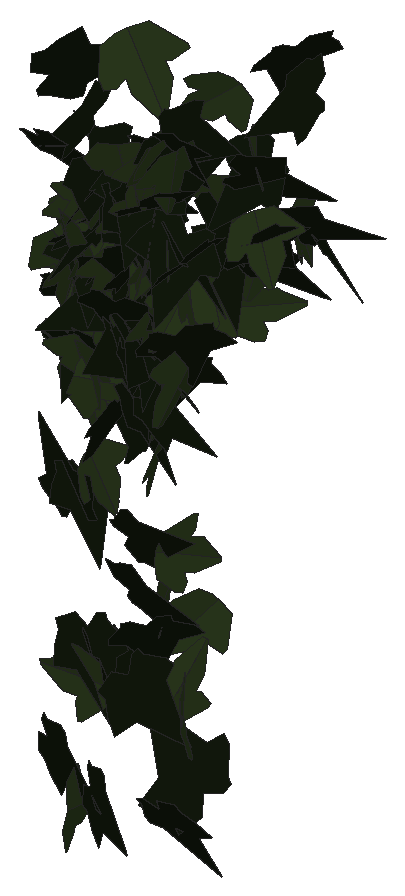
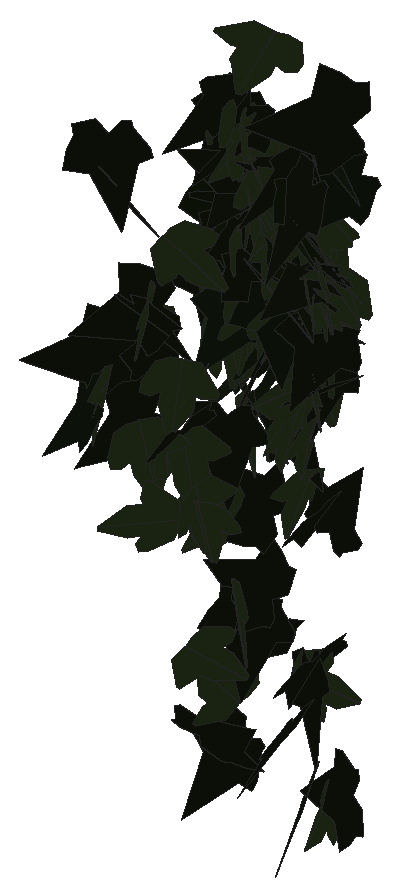
# SketchUp Ruby script. Lengths in inches.
U = 1.inch
M = Sketchup.active_model
def pt(a) = Geom::Point3d.new(a.map { |v| v * U })
def face(e, loops, mat)
  f = e.add_face(loops[0].map { |a| pt(a) })
  loops[1..].each { |l| e.add_face(l.map { |a| pt(a) }).erase! }
  f.material = f.back_material = mat if mat
  f
end
# faces: each face lists its corners as indices into pts; further lists are holes
def faces(e, pts, list, mat = nil) = list.each { |f| face(e, (f[0].is_a?(Array) ? f : [f]).map { |l| l.map { |i| pts[i] } }, mat) }
# xy, xz, yz: faces in a plane at the given z, y or x. An outline is a flat list of corners, or four numbers for a rectangle; further outlines are holes
def ring(l) = l.size == 4 ? [[l[0], l[1]], [l[2], l[1]], [l[2], l[3]], [l[0], l[3]]] : l.each_slice(2).to_a
def flat(e, list, mat, &to3) = list.each { |f| face(e, (f[0].is_a?(Array) ? f : [f]).map { |l| ring(l).map { |u, v| to3.(u, v) } }, mat) }
def xy(e, z, list, mat = nil) = flat(e, list, mat) { |x, y| [x, y, z] }
def xz(e, y, list, mat = nil) = flat(e, list, mat) { |x, z| [x, y, z] }
def yz(e, x, list, mat = nil) = flat(e, list, mat) { |y, z| [x, y, z] }
def lines(e, pts, list) = list.each { |a, b| e.add_line(pt(pts[a]), pt(pts[b])) }
# prism: a flat outline (further loops are holes) pulled along v
def prism(e, loops, v, mat = nil)
  f = face(e, loops, mat); d = Geom::Vector3d.new(v.map { |x| x * U })
  f.pushpull(f.normal.samedirection?(d) ? d.length : -d.length)
end
def box(e, o, s, mat = nil) = prism(e, [[o, [o[0] + s[0], o[1], o[2]], [o[0] + s[0], o[1] + s[1], o[2]], [o[0], o[1] + s[1], o[2]]]], [0, 0, s[2]], mat)
def at(x, y, z, deg = 0) = Geom::Transformation.translation(pt([x, y, z])) * Geom::Transformation.rotation(ORIGIN, Z_AXIS, deg.degrees)
def axes(o, x, y, z) = Geom::Transformation.new([*x, 0, *y, 0, *z, 0, *pt(o).to_a, 1])
def part(name) = M.definitions.add(name)
# library, detail: a bought-in or finely detailed component or shape, given as its bounding box
def library(name, o, s) = part(name).tap { |d| box(d.entities, o, s) }
def detail(e, o, s) = box(e.add_group.entities, o, s)
def put(e, d, t, mat = nil) = e.add_instance(d, t).tap { |i| i.material = mat if mat }
def group(e, t, mat = nil) = e.add_group.tap { |g| g.transformation = t; g.material = mat if mat }.entities
root = M.entities
M.materials.add("efeu1").color = [18, 25, 13]
M.materials.add("efeu2").color = [43, 57, 29]
c1 = part("ivyleaf_9")
p = [[1.54,2.16,1.25],[1.36,2.04,1.19],[-0.21,0.99,0.68],[-0.71,1.11,0.82],[-0.85,0.86,0.67],[-0.8,0.17,0.21],
  [-0.9,-0.01,0.1],[-0.67,-0.16,-0.02],[-0.08,-0.08,-0.05],[-0.03,-0.6,-0.4],[0.65,-0.88,-0.66],[0.83,-0.6,-0.49],
  [1.29,-0.42,-0.43],[1.8125,-0.07,-0.26],[1.21,0.44,0.15]]
faces(c1.entities,p,[[0,1,2,3,4,5,6,7,8,9,10,11,12,13,14]],"efeu1")
c2 = part("ivyleaf_10")
p = [[0,0.5,-0.03],[-0.0625,2.02,-0.43],[-0.19,2.01,-0.46],[-0.54,1.05,-0.29],[-0.52,0.625,-0.18],[-0.83,0.76,-0.28],
  [-1.16,0.64,-0.33],[-1.15,0.33,-0.24],[-0.77,-0.39,0.02],[-0.3,-0.51,0.16],[0.04,-0.48,0.23],[-0.02,2.01,-0.4375],
  [-0.06,2.01,-0.43],[0.04,-0.49,0.23],[0.67,-0.49,0.14],[1.38,0.36,-0.2],[1.375,0.51,-0.24],[0.81,0.65,-0.19],
  [0.62,0.59,-0.15],[0.6,1.09,-0.28],[0.5,1.23,-0.31]]
faces(c2.entities,p,[[0,1,2,3,4,5,6,7,8,9,10],[11,12,0,13,14,15,16,17,18,19,20]],"efeu2")
put(root,c1,axes([544.76,134.72,188.62],[0.26461,-0.49015,-0.62261],[-0.11295,0.62638,-0.54111],[0.7843,0.25557,0.13213]))
put(root,c1,axes([544.53,135.6,197.67],[-0.09645,-0.52638,0.59874],[0.11267,-0.60605,-0.51465],[0.78922,0.02219,0.14664]))
put(root,c1,axes([545.9,135.43,201.21],[-0.46865,-0.66084,-0.06581],[0.07755,0.02553,-0.80871],[0.65957,-0.47256,0.04833]))
put(root,c2,axes([543.35,135.14,201.56],[-0.61815,-0.37302,0.40934],[-0.34419,-0.22182,-0.7219],[0.43386,-0.70743,0.01051]))
put(root,c2,axes([543.34,134.95,187.91],[0.05962,-0.02944,-0.83382],[-0.8038,0.22209,-0.06531],[0.22369,0.80591,-0.01246]))
put(root,c1,axes([544.24,134.74,199.09],[0.5135,0.45053,-0.41731],[-0.39056,-0.1802,-0.67513],[-0.47391,0.63668,0.10421]))
put(root,c1,axes([545.73,134.73,185.15],[0.85129,0.12056,-0.12346],[-0.12249,-0.01554,-0.85979],[-0.12154,0.86006,0.00177]))
put(root,c2,axes([545.02,135.13,200.87],[0.77564,-0.25844,-0.09532],[-0.09055,0.02979,-0.81756],[0.26015,0.78091,-0.00036]))
put(root,c2,axes([543.06,135.12,197.1],[-0.62944,-0.37013,0.31975],[-0.27822,-0.15765,-0.73019],[0.40228,-0.68817,-0.0047]))
put(root,c1,axes([543.95,135.68,197.38],[0.32213,-0.46197,-0.56698],[0.30459,-0.47851,0.56294],[-0.66491,-0.44302,-0.01681]))
put(root,c2,axes([545.8,135.56,197.49],[0.11949,-0.7861,0.55869],[0.12562,-0.54548,-0.79438],[0.95619,0.1699,0.03454]))
put(root,c2,axes([545.8,135.11,203.51],[-0.11866,-0.8194,-0.02635],[0.01545,0.02439,-0.82787],[0.81968,-0.11908,0.01179]))
put(root,c2,axes([544.25,134.98,203.22],[-0.69949,-0.4216,-0.0796],[0.0593,0.05578,-0.81655],[0.42494,-0.7018,-0.01708]))
put(root,c2,axes([543,134.97,197.16],[-0.72287,0.30848,-0.06623],[0.05691,-0.03537,-0.78587],[-0.31034,-0.72504,0.01016]))
put(root,c2,axes([542.57,134.92,200.67],[-0.74013,0.35899,0.06304],[-0.05424,0.03261,-0.82258],[-0.36042,-0.74209,-0.00565]))
put(root,c2,axes([544.97,135.35,203.03],[-0.15827,-0.75081,0.27557],[-0.01987,-0.27714,-0.76649],[0.79954,-0.15551,0.0355]))
put(root,c1,axes([543.5,135.375,201.18],[-0.68086,0.24372,-0.34248],[0.24183,-0.30612,-0.69862],[-0.34382,-0.69796,0.18682]))
put(root,c1,axes([544.46,135.12,192.33],[0.6246,0.15303,-0.47673],[0.43965,0.19707,0.63928],[0.23958,-0.76063,0.06972]))
put(root,c1,axes([546.18,134.77,198.79],[0.42333,0.69725,-0.21629],[-0.10931,-0.18667,-0.81569],[-0.72179,0.4372,-0.00333]))
put(root,c2,axes([544.79,135.5625,201.25],[-0.20567,0.32932,-0.7003],[0.18555,-0.68249,-0.37544],[-0.75129,-0.25871,0.09899]))
put(root,c2,axes([545,135.23,203.39],[0.21388,-0.79503,0.01086],[0.01094,-0.0083,-0.82325],[0.79503,0.21399,0.00841]))
put(root,c2,axes([542.95,134.57,184.39],[0.09931,-0.29894,-0.80701],[-0.04553,0.8094,-0.30543],[0.8594,0.07743,0.07707]))
put(root,c1,axes([543.23,135.03,203.92],[-0.55428,0.61063,0.06662],[-0.09364,0.00469,-0.82204],[-0.60708,-0.55825,0.06596]))
put(root,c1,axes([544.67,135.52,202.45],[-0.48451,-0.62371,-0.1688],[0.13918,0.10529,-0.78854],[0.63098,-0.50215,0.04433]))
put(root,c1,axes([541.84,134.87,202.86],[0.8272,0.06653,-0.0089],[-0.01473,0.07252,-0.82661],[-0.06549,0.82406,0.07346]))
put(root,c2,axes([544.58,135.11,201.8],[-0.3463,-0.70029,-0.17635],[0.10079,0.1468,-0.78085],[0.71509,-0.35982,0.02465]))
put(root,c1,axes([544.1875,135.39,201.78],[0.26114,-0.7518,-0.13057],[-0.05401,0.11945,-0.79578],[0.76114,0.26641,-0.01167]))
put(root,c2,axes([543.8,135.39,199.96],[-0.18823,-0.77605,0.16166],[-0.03684,-0.15741,-0.79855],[0.79185,-0.1918,0.00128]))
put(root,c2,axes([544.62,135.24,200.5],[0.55391,-0.56546,-0.20766],[-0.1416,0.15197,-0.79154],[0.5855,0.5717,0.00502]))
put(root,c1,axes([542.5625,134.99,197.46],[0.66487,0.22568,-0.35782],[-0.33337,-0.13085,-0.70197],[-0.26044,0.74361,-0.01492]))
put(root,c2,axes([545.88,135.46,199.6],[0.46267,0.52111,-0.41546],[-0.28247,-0.30476,-0.69682],[-0.60363,0.54203,0.00764]))
put(root,c1,axes([542.46,135.18,192.63],[0.39249,-0.24506,0.67965],[-0.43984,0.53257,0.44603],[-0.57317,-0.5765,0.12313]))
put(root,c1,axes([543.84,134.82,200.17],[0.61538,0.5123,0.01662],[0.0124,0.01108,-0.80071],[-0.51242,0.6155,0.00058]))
put(root,c1,axes([544.33,135.39,196.07],[0.5133,-0.61052,0.01301],[0.00313,-0.01437,-0.7976],[0.61065,0.51326,-0.00685]))
put(root,c1,axes([543.28,135.01,184.8],[0.50992,-0.33187,-0.57273],[-0.48933,0.29789,-0.60828],[0.44578,0.70662,-0.01256]))
put(root,c1,axes([544.98,135.55,198.59],[-0.59767,-0.19423,-0.50469],[0.50881,0.0528,-0.62288],[0.18316,-0.78047,0.08346]))
put(root,c1,axes([542.59,135.55,193.17],[0.14743,-0.7677,-0.05262],[0.00797,0.0551,-0.78152],[0.76946,0.14653,0.01818]))
put(root,c2,axes([543.52,135.33,201.78],[-0.06262,-0.81239,-0.06941],[-0.0248,0.07148,-0.81424],[0.81497,-0.06024,-0.03012]))
put(root,c1,axes([543.46,135.09,201.9375],[-0.26081,0.76593,-0.10414],[0.04542,-0.09454,-0.80902],[-0.77164,-0.26444,-0.01242]))
put(root,c1,axes([545.07,135,196.48],[0.68894,-0.28627,-0.37646],[-0.20713,0.41535,-0.69491],[0.42517,0.66622,0.27147]))
put(root,c1,axes([541.54,135.51,185.375],[0.15811,0.00107,-0.85529],[0.84517,0.13322,0.15641],[0.1312,-0.85952,0.02318]))
put(root,c1,axes([544.27,135.34,199.3],[-0.15862,-0.08005,-0.94213],[-0.87716,-0.3442,0.17693],[-0.35301,0.89123,-0.01629]))
put(root,c2,axes([542.81,135.45,201.24],[-0.45591,-0.66819,0.06412],[0.04088,-0.105,-0.80359],[0.67002,-0.44826,0.09265]))
put(root,c2,axes([545.1,135.41,195.11],[0.36867,-0.7287,-0.08806],[-0.03604,0.08045,-0.81664],[0.73311,0.3704,0.00414]))
put(root,c2,axes([545.31,135.34,203.62],[-0.02715,-0.80702,-0.12925],[0.00679,0.1291,-0.80747],[0.81728,-0.02788,0.00242]))
put(root,c1,axes([543.4375,134.87,202.9],[0.2769,-0.24019,-0.80036],[-0.24828,0.78143,-0.32041],[0.79789,0.32652,0.17806]))
put(root,c2,axes([542.36,135.45,199.43],[0.05786,-0.79891,-0.00714],[-0.0036,0.00689,-0.801],[0.79894,0.05789,-0.00309]))
put(root,c2,axes([543.19,134.99,196.52],[-0.12595,-0.28137,-0.73434],[0.59291,0.45457,-0.27587],[0.51659,-0.59033,0.13758]))
put(root,c1,axes([542.71,135.58,188.86],[0.19102,-0.8108,-0.17875],[-0.02798,0.17702,-0.83289],[0.8298,0.19261,0.01306]))
put(root,c1,axes([546.13,134.92,200.74],[0.04295,0.79783,0.13048],[-0.02384,0.13186,-0.79841],[-0.80808,0.03851,0.03049]))
put(root,c1,axes([543.67,135.74,198.625],[-0.67641,-0.14968,0.385],[-0.37222,-0.09942,-0.69262],[0.1791,-0.77193,0.01455]))
put(root,c1,axes([543.67,135.48,195.65],[-0.32845,0.58445,-0.4236],[0.21599,-0.36448,-0.67037],[-0.68874,-0.39302,-0.00822]))
put(root,c1,axes([545.02,134.83,202.1],[0.51354,0.57418,0.22881],[0.02985,0.2741,-0.75481],[-0.61737,0.49086,0.15383]))
put(root,c2,axes([542.98,135.43,201.16],[-0.73219,-0.32756,0.14451],[-0.11964,-0.0862,-0.80158],[0.33743,-0.74132,0.02935]))
put(root,c2,axes([546.26,134.95,187.67],[-0.11509,0.06058,0.89347],[-0.72917,0.51661,-0.12895],[-0.51988,-0.738,-0.01693]))
put(root,c2,axes([545.04,135.53,198.75],[-0.02148,-0.80655,-0.001],[0.00434,0.00089,-0.80682],[0.80654,-0.02149,0.00431]))
put(root,c1,axes([543.05,135.53,201.16],[-0.73594,0.33106,-0.02115],[0.01592,-0.01618,-0.80694],[-0.33136,-0.73607,0.00822]))
put(root,c2,axes([542.07,135.31,199.89],[-0.56922,-0.41986,-0.41689],[0.39499,0.16106,-0.70152],[0.44052,-0.68693,0.09033]))
put(root,c1,axes([543.11,135.23,188.39],[0.43066,-0.00474,-0.7673],[-0.76671,-0.03747,-0.43009],[-0.03036,0.87909,-0.02247]))
put(root,c2,axes([542.65,135.65,199.71],[0.31981,-0.72349,0.08485],[0.02424,-0.08205,-0.79094],[0.72804,0.32054,-0.01093]))
put(root,c1,axes([542.85,135.72,200.14],[-0.49918,-0.51061,-0.35288],[0.2638,0.23537,-0.71375],[0.56183,-0.56419,0.0216]))
put(root,c1,axes([543.73,135.64,201.12],[0.37923,-0.70472,-0.05999],[0.02956,0.0838,-0.79759],[0.70665,0.37469,0.06555]))
put(root,c2,axes([544.88,135.64,200.29],[0.08786,-0.79549,0.02743],[0.01075,-0.02641,-0.80029],[0.79589,0.08817,0.00778]))
put(root,c2,axes([544.3,135.37,206.1],[0.68849,0.51649,0.42703],[0.35488,0.23836,-0.86045],[-0.56849,0.77431,-0.01996]))
put(root,c1,axes([544.38,135.66,197.65],[0.57336,-0.49432,0.26465],[0.22701,-0.14146,-0.75604],[0.5127,0.61545,0.03879]))
put(root,c2,axes([542.61,135.51,200.18],[0.50951,-0.57099,-0.2545],[-0.1545,0.20312,-0.76504],[0.60575,0.53209,0.01893]))
put(root,c2,axes([543.53,135.67,200.86],[0.58527,0.44455,-0.31867],[-0.28801,-0.1463,-0.73305],[-0.465,0.65015,0.05294]))
put(root,c1,axes([545.16,135.17,203.79],[0.72885,0.34667,-0.05581],[-0.0707,0.01892,-0.8057],[-0.34394,0.73074,0.04734]))
put(root,c1,axes([544.93,135.24,195.63],[-0.40944,0.54734,0.41119],[-0.23124,0.34039,-0.68335],[-0.64436,-0.46995,-0.01605]))
put(root,c1,axes([543.96,135.77,190.375],[0.38096,-0.32428,0.67991],[0.57767,-0.36322,-0.49691],[0.48345,0.68954,0.058]))
put(root,c2,axes([542.71,135.81,197.92],[0.55663,-0.13923,0.53905],[0.52586,-0.11887,-0.57371],[0.18285,0.76569,0.00895]))
put(root,c1,axes([542.34,136.1875,196.98],[-0.34954,-0.66942,0.19408],[0.1395,-0.27992,-0.71426],[0.68289,-0.28547,0.24525]))
put(root,c2,axes([544.99,135.16,203.09],[0.02214,-0.40999,-0.7123],[0.26679,0.67755,-0.3817],[0.77736,-0.22086,0.15129]))
put(root,c2,axes([542.27,135.61,199.57],[-0.70243,-0.27071,-0.23913],[0.25849,-0.01151,-0.74628],[0.25229,-0.74193,0.09883]))
put(root,c2,axes([542.27,135.74,199.51],[0.78773,0.02043,-0.01835],[-0.01837,0.00059,-0.78799],[-0.02041,0.78794,0.00107]))
put(root,c2,axes([545.92,135.52,199.86],[-0.17875,0.7869,0.03925],[-0.01318,0.03725,-0.80694],[-0.78777,-0.17917,0.0046]))
put(root,c2,axes([543.08,135.39,193.85],[0.02177,0.74231,0.25477],[-0.02274,0.25536,-0.74208],[-0.78448,0.0132,0.02858]))
put(root,c1,axes([544.74,135.27,201.78],[0.01017,0.00045,0.82155],[0.77709,0.26663,-0.00976],[-0.26662,0.77715,0.00287]))
put(root,c1,axes([545.12,135.6,200.67],[0.32098,0.53495,-0.50611],[-0.27075,-0.4277,-0.62379],[-0.68484,0.41982,0.00941]))
put(root,c1,axes([545.39,135.8,200.95],[0.59675,-0.53668,-0.01954],[-0.02181,0.00497,-0.8025],[0.53659,0.59705,-0.01089]))
put(root,c2,axes([544.38,135.71,198.14],[-0.56996,-0.52951,-0.176],[0.17594,0.06821,-0.77498],[0.52953,-0.5926,0.06806]))
put(root,c1,axes([543.61,135.49,200.21],[-0.36178,0.69928,0.12269],[-0.03986,0.11747,-0.7871],[-0.70884,-0.3635,-0.01835]))
put(root,c1,axes([545.42,135.22,204.09],[0.09008,0.03024,-0.81627],[-0.13863,0.80987,0.0147],[0.80498,0.13609,0.09387]))
put(root,c1,axes([546.2,135.66,185.54],[-0.88303,-0.16496,-0.3684],[-0.36271,-0.06456,0.8983],[-0.17712,0.95462,-0.00291]))
put(root,c1,axes([544.42,135.71,199.83],[-0.09351,0.73235,-0.30272],[-0.02642,-0.30753,-0.73583],[-0.79201,-0.07621,0.06029]))
put(root,c1,axes([544.36,135.6,199.24],[-0.47874,0.4472,0.46501],[-0.34618,0.31057,-0.65508],[-0.54441,-0.59074,0.00763]))
put(root,c1,axes([544.64,135.53,189.67],[0.39455,0.673,-0.20865],[-0.12948,-0.1658,-0.77966],[-0.6926,0.41439,0.0269]))
put(root,c2,axes([542.52,135.9375,197.45],[0.53088,-0.57852,-0.03027],[0.01648,0.05612,-0.78359],[0.57907,0.52878,0.05005]))
put(root,c1,axes([544.05,135.64,197.55],[0.45583,-0.39345,-0.52624],[-0.38581,0.35818,-0.60197],[0.53187,0.59701,0.01435]))
put(root,c1,axes([541.84,135.29,204.54],[0.38876,0.19969,0.83467],[0.70564,0.44717,-0.43565],[-0.48848,0.80489,0.03495]))
put(root,c1,axes([542.51,135.31,200.26],[0.52328,0.48237,0.35709],[0.1466,0.35668,-0.69664],[-0.58198,0.52356,0.1456]))
put(root,c2,axes([542.57,135.86,195.77],[-0.1436,0.77613,-0.04261],[0.00307,-0.04276,-0.78928],[-0.77729,-0.14355,0.00475]))
put(root,c2,axes([545.52,135.34,192.14],[0.02531,0.28221,0.75815],[0.01585,0.7582,-0.28276],[-0.80882,0.02369,0.01819]))
put(root,c2,axes([545.05,135.78,198.28],[-0.88711,0.24227,0.29678],[-0.2867,0.07669,-0.9196],[-0.25411,-0.93229,0.00147]))
put(root,c1,axes([542.0625,135.64,198.67],[0.59385,0.51418,-0.05023],[-0.02987,-0.04222,-0.78542],[-0.51576,0.59447,-0.01234]))
put(root,c2,axes([543.57,135.84,198.87],[-0.0545,0.76435,0.1995],[0.00781,0.20049,-0.766],[-0.78992,-0.05076,-0.02134]))
put(root,c1,axes([544.82,135.6,198.42],[0.69007,0.41373,-0.01781],[-0.13868,0.19826,-0.76756],[-0.39021,0.66122,0.24129]))
put(root,c1,axes([543.58,135.8,199.1],[0.25382,0.72266,-0.20686],[-0.22571,-0.13499,-0.74852],[-0.717,0.29832,0.16241]))
put(root,c1,axes([542.56,135.91,202.71],[0.82968,-0.09375,-0.44782],[-0.44071,0.08533,-0.83438],[0.1229,0.93895,0.03111]))
put(root,c2,axes([542.89,135.88,196.27],[0.23207,0.64421,0.40094],[0.1026,0.38878,-0.68406],[-0.75182,0.25191,0.03041]))
put(root,c2,axes([544.52,136.34,190.45],[0.47847,-0.56999,-0.45075],[-0.21606,0.4037,-0.73983],[0.69382,0.51879,0.08046]))
put(root,c2,axes([544.83,136.16,187.4],[0.30523,0.55657,-0.56846],[0.29536,0.48607,0.63449],[0.7387,-0.42432,-0.01881]))
put(root,c2,axes([542.5625,136.62,196.25],[-0.10226,0.77125,-0.0598],[0.03269,-0.05596,-0.7776],[-0.77288,-0.10441,-0.02497]))
put(root,c1,axes([542.5,136.78,187.64],[0.48801,-0.52714,-0.46174],[-0.22928,0.4116,-0.71222],[0.6622,0.53098,0.09369]))
put(root,c2,axes([544.86,137.55,189.3],[0.35292,0.39946,-0.61544],[-0.45936,-0.41223,-0.53098],[-0.57212,0.5774,0.04668]))
put(root,c1,axes([544.01,137.43,196.21],[0.4279,0.52522,-0.40944],[-0.31293,-0.27103,-0.6747],[-0.58785,0.52658,0.06112]))
put(root,c2,axes([545.16,139.21,199.6],[0.49399,0.60753,0.18061],[0.10539,0.14707,-0.78295],[-0.62498,0.505,0.01073]))
put(root,c1,axes([546.51,139.67,203.66],[-0.77602,0.29218,0.09392],[-0.08813,0.03248,-0.8292],[-0.29398,-0.78101,0.00065]))
put(root,c1,axes([545.1,139.12,199.14],[0.39613,0.68525,0.1331],[0.06236,0.11769,-0.79149],[-0.69526,0.40098,0.00485]))
put(root,c2,axes([543.54,140.01,202.53],[0.43091,0.30587,-0.61086],[-0.66187,0.00806,-0.46287],[-0.16918,0.74751,0.25495]))
put(root,c1,axes([545.92,139.78,204.71],[0.10339,0.7596,-0.27697],[-0.08448,-0.26755,-0.76529],[-0.80409,0.12577,0.04479]))
put(root,c1,axes([544.46,140.45,200.64],[-0.82387,-0.06194,-0.06901],[0.06815,0.01391,-0.82615],[0.06288,-0.82664,-0.00873]))
put(root,c1,axes([542.91,140.79,198.32],[0.02076,-0.59408,0.51555],[0.0231,-0.51504,-0.59443],[0.78625,0.03082,0.00386]))
put(root,c1,axes([544.24,139.86,200.48],[0.66091,0.17443,0.45446],[0.44172,0.10709,-0.6835],[-0.20454,0.7949,-0.00764]))
put(root,c2,axes([542.88,140.52,197.18],[-0.4257,-0.68459,0.09379],[-0.03905,-0.08616,-0.80606],[0.68988,-0.42731,0.01226]))
put(root,c1,axes([542.85,140.7,197.74],[0.1185,-0.76308,-0.14403],[-0.04279,0.13906,-0.77195],[0.77537,0.1243,-0.02059]))
put(root,c2,axes([542.26,140.71,195.97],[-0.12974,-0.77331,0.17823],[0.18642,-0.20525,-0.75481],[0.77138,-0.08047,0.21239]))
put(root,c2,axes([542.2,140.65,195.6],[0.78429,0.1598,-0.01715],[-0.0138,-0.01817,-0.80026],[-0.16013,0.78426,-0.01505]))
put(root,c2,axes([544.15,140.41,200.91],[-0.42972,0.65069,0.14845],[-0.09785,0.11322,-0.77955],[-0.66019,-0.44031,0.01892]))
put(root,c2,axes([542.92,140.73,199.34],[-0.71322,-0.33296,-0.03075],[0.0249,0.01934,-0.78708],[0.33345,-0.71362,-0.00699]))
put(root,c1,axes([545.09,140.58,199.07],[0.60626,-0.02714,0.55158],[0.54594,0.15292,-0.59253],[-0.08325,0.80524,0.13112]))
put(root,c1,axes([543.95,140.57,197.76],[0.75876,0.20956,0.20212],[0.19618,0.04888,-0.78715],[-0.21512,0.78369,-0.00495]))
put(root,c2,axes([543.71,141.24,197.48],[-0.62481,-0.46802,0.23312],[-0.20113,-0.12017,-0.78031],[0.48264,-0.65596,-0.02338]))
put(root,c2,axes([544.8,141.33,198.78],[-0.32012,0.68131,0.32435],[-0.22006,0.25272,-0.74804],[-0.72177,-0.37922,0.08422]))
put(root,c1,axes([544.68,141.9,198.375],[0.70477,-0.40615,-0.05695],[-0.06056,0.00892,-0.81312],[0.40563,0.70701,-0.02246]))
put(root,c2,axes([542.85,141.47,195.5],[0.00143,-0.01779,0.80228],[0.36014,0.71696,0.01526],[-0.71712,0.36003,0.00926]))
